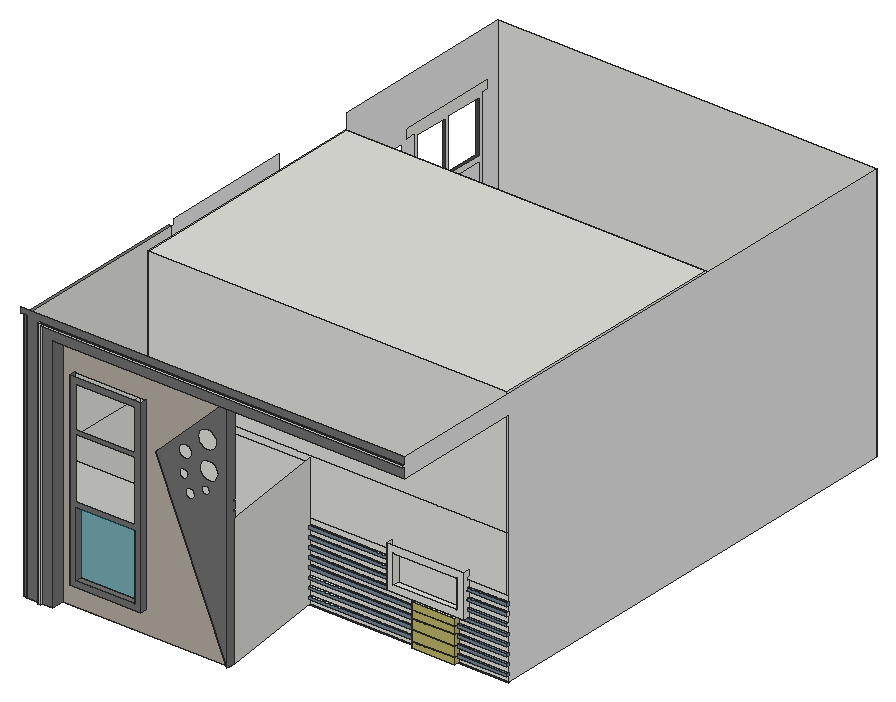
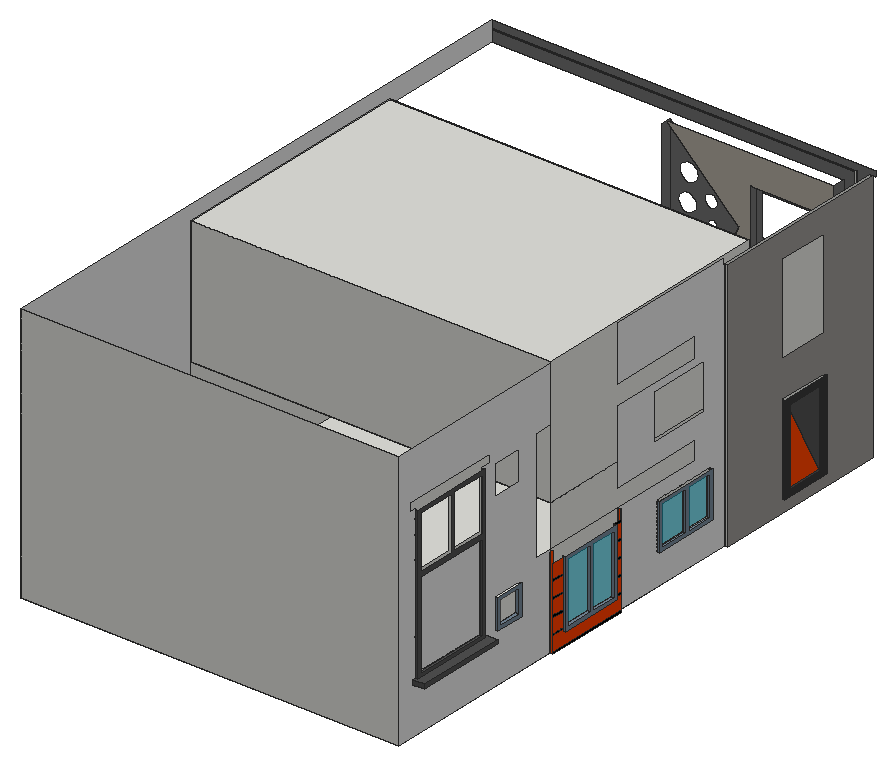
# SketchUp Ruby script. Lengths in inches.
U = 1.inch
M = Sketchup.active_model
def pt(a) = Geom::Point3d.new(a.map { |v| v * U })
def face(e, loops, mat)
  f = e.add_face(loops[0].map { |a| pt(a) })
  loops[1..].each { |l| e.add_face(l.map { |a| pt(a) }).erase! }
  f.material = f.back_material = mat if mat
  f
end
# faces: each face lists its corners as indices into pts; further lists are holes
def faces(e, pts, list, mat = nil) = list.each { |f| face(e, (f[0].is_a?(Array) ? f : [f]).map { |l| l.map { |i| pts[i] } }, mat) }
# xy, xz, yz: faces in a plane at the given z, y or x. An outline is a flat list of corners, or four numbers for a rectangle; further outlines are holes
def ring(l) = l.size == 4 ? [[l[0], l[1]], [l[2], l[1]], [l[2], l[3]], [l[0], l[3]]] : l.each_slice(2).to_a
def flat(e, list, mat, &to3) = list.each { |f| face(e, (f[0].is_a?(Array) ? f : [f]).map { |l| ring(l).map { |u, v| to3.(u, v) } }, mat) }
def xy(e, z, list, mat = nil) = flat(e, list, mat) { |x, y| [x, y, z] }
def xz(e, y, list, mat = nil) = flat(e, list, mat) { |x, z| [x, y, z] }
def yz(e, x, list, mat = nil) = flat(e, list, mat) { |y, z| [x, y, z] }
def lines(e, pts, list) = list.each { |a, b| e.add_line(pt(pts[a]), pt(pts[b])) }
# prism: a flat outline (further loops are holes) pulled along v
def prism(e, loops, v, mat = nil)
  f = face(e, loops, mat); d = Geom::Vector3d.new(v.map { |x| x * U })
  f.pushpull(f.normal.samedirection?(d) ? d.length : -d.length)
end
def box(e, o, s, mat = nil) = prism(e, [[o, [o[0] + s[0], o[1], o[2]], [o[0] + s[0], o[1] + s[1], o[2]], [o[0], o[1] + s[1], o[2]]]], [0, 0, s[2]], mat)
def at(x, y, z, deg = 0) = Geom::Transformation.translation(pt([x, y, z])) * Geom::Transformation.rotation(ORIGIN, Z_AXIS, deg.degrees)
def axes(o, x, y, z) = Geom::Transformation.new([*x, 0, *y, 0, *z, 0, *pt(o).to_a, 1])
def part(name) = M.definitions.add(name)
# library, detail: a bought-in or finely detailed component or shape, given as its bounding box
def library(name, o, s) = part(name).tap { |d| box(d.entities, o, s) }
def detail(e, o, s) = box(e.add_group.entities, o, s)
def put(e, d, t, mat = nil) = e.add_instance(d, t).tap { |i| i.material = mat if mat }
def group(e, t, mat = nil) = e.add_group.tap { |g| g.transformation = t; g.material = mat if mat }.entities
root = M.entities
M.materials.add("[0024_OrangeRed]").color = [255, 69, 0]
M.materials.add("[0057_DarkKhaki]").color = [189, 183, 107]
M.materials.add("[0110_LightSlateGray]").color = [119, 136, 153]
M.materials.add("[0135_DarkGray]").color = [81, 81, 81]
M.materials.add("[Color B05]").color = [255, 63, 0]
M.materials.add("[Color M05]").color = [114, 114, 114]
M.materials.add("[Color M07]").color = [58, 58, 58]
M.materials.add("[Color M09]").color = [0, 0, 0]
M.materials.add("[Concrete Aggregate Smoke]").color = [154, 150, 148]
M.materials.add("[Polished Concrete Old]").color = [229, 229, 229]
M.materials.add("[Stone Masonry Multi]").color = [182, 175, 164]
M.materials.add("[Translucent Glass Gray]").color = [128, 128, 128]
M.materials["[Translucent Glass Gray]"].alpha = 0.5
M.materials.add("[Translucent Glass Tinted]").color = [4, 119, 142]
M.materials["[Translucent Glass Tinted]"].alpha = 0.48
M.materials.add("[Translucent Glass Tinted]1").color = [8, 201, 241]
M.materials["[Translucent Glass Tinted]1"].alpha = 0.48
xy(root,0,[[15,20,18,175.3125],[18,20,18,563,378,563,378,125.9375,27,125.9375,27,20],[27,20,27,125.9375,188.34,125.9375,201.375,20],[15,302.14,18,382.63]])
xy(root,0,[[289.59,120.9375,330.37,125.9375]],"[0057_DarkKhaki]")
xy(root,0,[[30.46,0,30.46,2,18,2,18,20,201.375,20,201.375,14,42.91,14,42.91,2,32.7,2,32.7,0],[15,2,18,20]],"[Color M05]")
xy(root,4.9,[[188.34,123.9375,289.59,125.9375],[330.37,123.9375,363.6875,125.9375],[363.6875,123.9375,378,125.9375]],"[0110_LightSlateGray]")
xy(root,5.67,[[289.59,120.9375,330.37,122.9375]])
xy(root,6.45,[[289.59,120.9375,330.37,122.9375]],"[0057_DarkKhaki]")
xy(root,7.97,[[188.34,123.9375,289.59,125.9375]])
xy(root,7.97,[[330.37,123.9375,378,125.9375]],"[0110_LightSlateGray]")
xy(root,13.12,[[12,60.99,15,110.86]],"[Color M07]")
xy(root,13.47,[[188.34,123.9375,289.59,125.9375],[330.37,123.9375,363.6875,125.9375],[363.6875,123.9375,378,125.9375]],"[0110_LightSlateGray]")
xy(root,15.375,[[12,310.47,15,371.75]],"[0110_LightSlateGray]")
xy(root,15.48,[[289.59,120.9375,330.37,122.9375]])
xy(root,16.27,[[289.59,120.9375,330.37,122.9375]],"[0057_DarkKhaki]")
xy(root,16.53,[[188.34,123.9375,289.59,125.9375]])
xy(root,16.53,[[330.37,123.9375,378,125.9375]],"[0110_LightSlateGray]")
xy(root,18.375,[[12,313.47,15,338.88],[12,341.11,15,368.75]],"[0110_LightSlateGray]")
xy(root,19.12,[[12,66.99,15,104.86]],"[Color M07]")
xy(root,20.43,[[53.9,8,121.9,14]],"[Color M05]")
xy(root,22.03,[[188.34,123.9375,289.59,125.9375],[330.37,123.9375,363.6875,125.9375],[363.6875,123.9375,378,125.9375]],"[0110_LightSlateGray]")
xy(root,25.09,[[188.34,123.9375,289.59,125.9375]])
xy(root,25.09,[[330.37,123.9375,378,125.9375]],"[0110_LightSlateGray]")
xy(root,25.29,[[289.59,120.9375,330.37,122.9375]])
xy(root,26.08,[[289.59,120.9375,330.37,122.9375]],"[0057_DarkKhaki]")
xy(root,26.43,[[59.9,8,115.9,14]],"[Color M05]")
xy(root,30.59,[[188.34,123.9375,289.59,125.9375],[330.37,123.9375,363.6875,125.9375],[363.6875,123.9375,378,125.9375]],"[0110_LightSlateGray]")
xy(root,30.87,[[15,192.9,18,256.21]],"[0110_LightSlateGray]")
xy(root,32.17,[[289.59,120.9375,330.37,122.9375]])
xy(root,32.95,[[289.59,120.9375,330.37,122.9375]],"[0057_DarkKhaki]")
xy(root,33.66,[[188.34,123.9375,289.59,125.9375]])
xy(root,33.66,[[330.37,123.9375,378,125.9375]],"[0110_LightSlateGray]")
xy(root,33.87,[[15,195.9,18,221.52],[15,224.56,18,253.21]],"[0110_LightSlateGray]")
xy(root,39.15,[[289.59,120.9375,330.37,123.9375],[289.59,123.9375,330.37,125.9375]])
xy(root,39.15,[[188.34,123.9375,289.59,125.9375],[330.37,123.9375,363.6875,125.9375],[363.6875,123.9375,378,125.9375]],"[0110_LightSlateGray]")
xy(root,42.22,[[266.69,119.9375,339.4,123.9375],[188.34,123.9375,266.69,125.9375],[266.69,123.9375,339.4,125.9375]])
xy(root,42.22,[[339.4,123.9375,378,125.9375]],"[0110_LightSlateGray]")
xy(root,45.35,[[6,459.92,18,547.29]],"[0135_DarkGray]")
xy(root,47.72,[[188.34,123.9375,266.69,125.9375],[339.4,123.9375,363.6875,125.9375],[363.6875,123.9375,378,125.9375]],"[0110_LightSlateGray]")
xy(root,48.22,[[272.69,119.9375,333.4,125.9375]])
xy(root,48.55,[[15,420.33,18,448.89]],"[0110_LightSlateGray]")
xy(root,49.6,[[15,463.73,18,543.73]])
xy(root,49.6,[[6,459.92,18,459.92,18,463.73,15,463.73,15,543.73,18,543.73,18,547.29,6,547.29]],"[0135_DarkGray]")
xy(root,50.78,[[188.34,123.9375,266.69,125.9375]])
xy(root,50.78,[[339.4,123.9375,378,125.9375]],"[0110_LightSlateGray]")
xy(root,51.55,[[15,423.33,18,445.89]],"[0110_LightSlateGray]")
xy(root,52.6,[[15,466.73,18,540.73]],"[0135_DarkGray]")
xy(root,56.28,[[188.34,123.9375,266.69,125.9375],[339.4,123.9375,363.6875,125.9375],[363.6875,123.9375,378,125.9375]],"[0110_LightSlateGray]")
xy(root,59.34,[[188.34,123.9375,266.69,125.9375]])
xy(root,59.34,[[339.4,123.9375,378,125.9375]],"[0110_LightSlateGray]")
xy(root,64.84,[[188.34,123.9375,266.69,125.9375],[339.4,123.9375,363.6875,125.9375],[363.6875,123.9375,378,125.9375]],"[0110_LightSlateGray]")
xy(root,67.91,[[188.34,123.9375,266.69,125.9375]])
xy(root,67.91,[[339.4,123.9375,378,125.9375]],"[0110_LightSlateGray]")
xy(root,71.62,[[15,195.9,18,221.52],[15,224.56,18,253.21]],"[0110_LightSlateGray]")
xy(root,120,[[27,134.9375,369,371]])
xy(root,240,[[27,134.9375,369,371]])
xz(root,0,[[30.46,0,32.7,0,32.7,238.03,378,238.03,378,239.39,30.46,239.39]])
xz(root,2,[[18,0,30.46,0,30.46,239.39,378,239.39,378,246,12,246,12,240.8125,18,240.8125],[15,0,18,240.8125],[32.7,0,42.91,0,42.91,227.53,378,227.53,378,238.03,32.7,238.03]],"[Color M05]")
xz(root,8,[[[53.9,20.43,121.9,200.12],[59.9,26.43,115.9,89.01],[59.9,93.35,115.9,151.59],[59.9,155.16,115.9,194.12]]],"[Color M05]")
xz(root,11,[[[201.375,0,201.375,227.53,133.54,160.93],[182.83,179.81,180.54,180.11,178.4,181,176.56,182.41,175.15,184.25,174.26,186.39,173.96,188.68,174.26,190.98,175.15,193.12,176.56,194.96,178.4,196.37,180.54,197.26,182.83,197.56,185.13,197.26,187.27,196.37,189.11,194.96,190.52,193.12,191.41,190.98,191.71,188.68,191.41,186.39,190.52,184.25,189.11,182.41,187.27,181,185.13,180.11],[184.53,153.64,182.23,153.94,180.1,154.83,178.27,156.24,176.86,158.07,175.97,160.2,175.67,162.49,175.97,164.79,176.86,166.92,178.27,168.75,180.1,170.16,182.23,171.05,184.53,171.35,186.82,171.05,188.95,170.16,190.79,168.75,192.19,166.92,193.08,164.79,193.38,162.49,193.08,160.2,192.19,158.07,190.79,156.24,188.95,154.83,186.82,153.94],[161.99,165.1,160.37,165.31,158.86,165.93,157.57,166.93,156.58,168.22,155.95,169.73,155.74,171.35,155.95,172.96,156.58,174.47,157.57,175.77,158.86,176.76,160.37,177.38,161.99,177.6,163.61,177.38,165.11,176.76,166.41,175.77,167.4,174.47,168.03,172.96,168.24,171.35,168.03,169.73,167.4,168.22,166.41,166.93,165.11,165.93,163.61,165.31],[166.47,132.54,165.33,132.69,164.28,133.13,163.375,133.83,162.68,134.73,162.24,135.79,162.09,136.92,162.24,138.05,162.68,139.11,163.375,140.01,164.28,140.71,165.33,141.14,166.47,141.29,167.6,141.14,168.65,140.71,169.5625,140.01,170.26,139.11,170.69,138.05,170.84,136.92,170.69,135.79,170.26,134.73,169.5625,133.83,168.65,133.13,167.6,132.69],[160.62,147.68,159.54,147.83,158.53,148.24,157.66,148.91,156.99,149.78,156.58,150.79,156.43,151.87,156.58,152.95,156.99,153.96,157.66,154.83,158.53,155.5,159.54,155.92,160.62,156.06,161.7,155.92,162.71,155.5,163.58,154.83,164.25,153.96,164.67,152.95,164.81,151.87,164.67,150.79,164.25,149.78,163.58,148.91,162.71,148.24,161.7,147.83],[181.03,140.83,180.03,140.97,179.09,141.35,178.29,141.97,177.67,142.77,177.29,143.71,177.15,144.71,177.29,145.71,177.67,146.65,178.29,147.45,179.09,148.0625,180.03,148.45,181.03,148.58,182.03,148.45,182.97,148.0625,183.77,147.45,184.39,146.65,184.77,145.71,184.9,144.71,184.77,143.71,184.39,142.77,183.77,141.97,182.97,141.35,182.03,140.97]]],"[Color M05]")
xz(root,14,[[[42.91,0,201.375,0,133.54,160.93,201.375,227.53,42.91,227.53],[53.9,20.43,121.9,200.12]]],"[Stone Masonry Multi]")
xz(root,14,[[59.9,26.43,115.9,89.01]],"[Translucent Glass Tinted]")
xz(root,20,[[27,0,201.375,120]])
xz(root,60.99,[[12,13.12,15,97.99]],"[Color M07]")
xz(root,66.99,[[12,19.12,15,91.99]],"[Color M07]")
xz(root,104.86,[[12,19.12,15,91.99]],"[Color M07]")
xz(root,110.86,[[12,13.12,15,97.99]],"[Color M07]")
xz(root,119.9375,[[[266.69,42.22,339.4,81.97],[272.69,48.22,333.4,75.97]]])
xz(root,120.9375,[[289.59,0,330.37,5.67],[289.59,6.45,330.37,15.48],[289.59,16.27,330.37,25.29],[289.59,26.08,330.37,32.17],[289.59,32.95,330.37,39.15]],"[0057_DarkKhaki]")
xz(root,122.9375,[[289.59,5.67,330.37,6.45],[289.59,15.48,330.37,16.27],[289.59,25.29,330.37,26.08],[289.59,32.17,330.37,32.95]],"[0057_DarkKhaki]")
xz(root,123.9375,[[188.34,4.9,289.59,7.97],[330.37,4.9,378,7.97],[188.34,13.47,289.59,16.53],[330.37,13.47,378,16.53],[188.34,22.03,289.59,25.09],
  [330.37,22.03,378,25.09],[188.34,30.59,289.59,33.66],[330.37,30.59,378,33.66],[188.34,39.15,378,42.22],[188.34,47.72,266.69,50.78],
  [339.4,47.72,378,50.78],[188.34,56.28,266.69,59.34],[339.4,56.28,378,59.34],[188.34,64.84,266.69,67.91],[339.4,64.84,378,67.91]],"[0110_LightSlateGray]")
xz(root,125.9375,[[188.34,-0.59,378,0],[27,0,188.34,120],[188.34,0,289.59,4.9],[330.37,0,378,4.9],[188.34,4.9,289.59,7.97],
  [330.37,4.9,378,7.97],[188.34,7.97,289.59,13.47],[330.37,7.97,378,13.47],[188.34,13.47,289.59,16.53],[330.37,13.47,378,16.53],
  [188.34,16.53,289.59,22.03],[330.37,16.53,378,22.03],[188.34,22.03,289.59,25.09],[330.37,22.03,378,25.09],[188.34,25.09,289.59,30.59],
  [330.37,25.09,378,30.59],[188.34,30.59,289.59,33.66],[330.37,30.59,378,33.66],[188.34,33.66,289.59,39.15],[330.37,33.66,378,39.15],
  [188.34,39.15,378,42.22],[188.34,42.22,266.69,47.72],[339.4,42.22,378,47.72],[188.34,47.72,266.69,50.78],[272.69,48.22,333.4,75.97],
  [188.34,50.78,266.69,56.28],[339.4,50.78,378,56.28],[188.34,56.28,266.69,59.34],[339.4,56.28,378,59.34],[188.34,59.34,266.69,64.84],
  [339.4,59.34,378,64.84],[188.34,64.84,266.69,67.91],[339.4,64.84,378,67.91],[188.34,67.91,266.69,73.4],[339.4,67.91,378,73.4]])
xz(root,134.9375,[[27,0,369,120],[27,120,369,240]])
xz(root,175.3125,[[15,0,18,240.8125]])
xz(root,192.9,[[15,30.87,18,74.62]],"[0110_LightSlateGray]")
xz(root,195.9,[[15,33.87,18,71.62]],"[0110_LightSlateGray]")
xz(root,221.52,[[15,33.87,18,71.62]],"[0110_LightSlateGray]")
xz(root,224.56,[[15,33.87,18,71.62]],"[0110_LightSlateGray]")
xz(root,253.21,[[15,33.87,18,71.62]],"[0110_LightSlateGray]")
xz(root,256.21,[[15,30.87,18,74.62]],"[0110_LightSlateGray]")
xz(root,302.14,[[15,0,18,88.11]],"[0024_OrangeRed]")
xz(root,310.47,[[12,15.375,15,17.625],[12,17.625,15,79.125]],"[0110_LightSlateGray]")
xz(root,313.47,[[12,18.375,15,76.125]],"[0110_LightSlateGray]")
xz(root,338.88,[[12,18.375,15,76.125]],"[0110_LightSlateGray]")
xz(root,341.11,[[12,18.375,15,76.125]],"[0110_LightSlateGray]")
xz(root,368.75,[[12,18.375,15,76.125]],"[0110_LightSlateGray]")
xz(root,371,[[27,120,369,240]])
xz(root,371.75,[[12,15.375,15,79.125]],"[0110_LightSlateGray]")
xz(root,382.63,[[15,0,18,88.11]],"[0024_OrangeRed]")
xz(root,420.33,[[15,48.55,18,77.11]],"[0110_LightSlateGray]")
xz(root,423.33,[[15,51.55,18,74.11]],"[0110_LightSlateGray]")
xz(root,445.89,[[15,51.55,18,74.11]],"[0110_LightSlateGray]")
xz(root,448.89,[[15,48.55,18,77.11]],"[0110_LightSlateGray]")
xz(root,459.92,[[6,45.35,18,49.6]],"[0135_DarkGray]")
xz(root,463.73,[[15,49.6,18,193.1]],"[0135_DarkGray]")
xz(root,466.73,[[15,52.6,18,135.41]],"[0135_DarkGray]")
xz(root,540.73,[[15,52.6,18,135.41]],"[0135_DarkGray]")
xz(root,543.73,[[15,49.6,18,193.1]],"[0135_DarkGray]")
xz(root,547.29,[[6,45.35,18,49.6]],"[0135_DarkGray]")
xz(root,563,[[18,0,378,246]])
yz(root,6,[[459.92,45.35,547.29,49.6]],"[0135_DarkGray]")
yz(root,12,[[[310.47,15.375,371.75,79.125],[341.11,18.375,368.75,76.125],[313.47,18.375,338.88,76.125]]],"[0110_LightSlateGray]")
yz(root,12,[[[60.99,13.12,110.86,97.99],[66.99,19.12,104.86,91.99]]],"[Color M07]")
yz(root,15,[[66.99,19.12,104.86,91.99,104.86,19.12]],"[0024_OrangeRed]")
yz(root,15,[[[192.9,30.87,256.21,74.62],[224.56,33.87,253.21,71.62],[195.9,33.87,221.52,71.62]],[[420.33,48.55,448.89,77.11],[423.33,51.55,445.89,74.11]]],"[0110_LightSlateGray]")
yz(root,15,[[66.99,19.12,66.99,91.99,104.86,91.99],[[463.73,49.6,543.73,193.1],[466.73,52.6,540.73,135.41],[503.73,139.68,540.73,190.1],[466.73,139.68,500.63,190.1]]],"[0135_DarkGray]")
yz(root,15,[[302.36,2.25,382.63,15.375],[302.36,17.625,310.47,30.75],[371.75,17.625,382.63,30.75],[302.36,33,310.47,46.125],[371.75,33,382.63,46.125],
  [302.36,48.375,310.47,61.5],[371.75,48.375,382.63,61.5],[302.36,63.75,310.47,76.875],[371.75,63.75,382.63,76.875]],"[Color B05]")
yz(root,15,[[302.14,0,302.14,88.11,302.36,88.11,302.36,79.125,310.47,79.125,310.47,76.875,302.36,76.875,302.36,63.75,310.47,63.75,310.47,61.5,302.36,61.5,302.36,48.375,310.47,48.375,310.47,46.125,302.36,46.125,302.36,33,310.47,33,310.47,30.75,302.36,30.75,302.36,17.625,310.47,17.625,310.47,15.375,302.36,15.375,302.36,2.25,382.63,2.25,382.63,0],[371.75,15.375,382.63,17.625],[371.75,30.75,382.63,33],[371.75,46.125,382.63,48.375],[371.75,61.5,382.63,63.75]],"[Color M09]")
yz(root,15,[[[2,0,175.3125,240.8125],[60.99,132.49,110.86,217.37],[60.99,13.12,110.86,97.99]]],"[Concrete Aggregate Smoke]")
yz(root,15,[[313.47,18.375,338.88,76.125],[341.11,18.375,368.75,76.125]],"[Translucent Glass Tinted]1")
yz(root,18,[[2,0,175.3125,240.8125],[302.14,0,382.63,88.11],[[192.9,30.87,256.21,74.62],[224.56,33.87,253.21,71.62],[195.9,33.87,221.52,71.62]],[[463.73,49.6,463.73,193.1,453.79,193.1,453.79,201.17,549.98,201.17,549.98,193.1,543.73,193.1,543.73,49.6],[466.73,52.6,540.73,135.41],[503.73,139.68,540.73,190.1],[466.73,139.68,500.63,190.1]]])
yz(root,18,[[[175.3125,0,175.3125,240.8125,177.0625,240.8125,177.0625,246,302.36,246,302.36,194.23,209.95,194.23,209.95,174.92,302.36,174.92,302.36,105.46,209.95,105.46,209.95,88.11,302.14,88.11,302.14,0],[192.9,30.87,256.21,74.62],[200.12,124.92,258.87,168.42]],[[382.63,0,382.63,88.11,399.82,88.11,399.82,194.23,382.63,194.23,382.63,246,563,246,563,0],[459.92,45.35,547.29,45.35,547.29,49.6,543.73,49.6,543.73,193.1,549.98,193.1,549.98,201.17,453.79,201.17,453.79,193.1,463.73,193.1,463.73,49.6,459.92,49.6],[420.33,161.99,448.89,190.55],[420.33,48.55,448.89,77.11]],[466.73,52.6,540.73,135.41]],"[Polished Concrete Old]")
yz(root,18,[[423.33,51.55,445.89,74.11]],"[Translucent Glass Gray]")
yz(root,18,[[195.9,33.87,221.52,71.62],[224.56,33.87,253.21,71.62]],"[Translucent Glass Tinted]1")
yz(root,27,[[20,0,125.9375,120],[134.9375,0,371,120],[134.9375,120,371,240]])
yz(root,30.46,[[0,0,2,239.39]])
yz(root,32.7,[[0,0,2,238.03]])
yz(root,42.91,[[2,0,14,227.53]],"[Color M05]")
yz(root,53.9,[[8,20.43,14,200.12]],"[Color M05]")
yz(root,59.9,[[8,26.43,14,89.01]],"[Color M05]")
yz(root,115.9,[[8,26.43,14,89.01]],"[Color M05]")
yz(root,121.9,[[8,20.43,14,200.12]],"[Color M05]")
yz(root,188.34,[[123.9375,4.9,125.9375,7.97],[123.9375,13.47,125.9375,16.53],[123.9375,22.03,125.9375,25.09],[123.9375,30.59,125.9375,33.66],[123.9375,39.15,125.9375,42.22],
  [123.9375,47.72,125.9375,50.78],[123.9375,56.28,125.9375,59.34],[123.9375,64.84,125.9375,67.91]])
yz(root,201.375,[[11,0,20,0,20,130.4,18,130.4,18,131.88,20,131.88,20,139.21,18,139.21,18,140.7,20,140.7,20,227.53,11,227.53]],"[Color M05]")
yz(root,266.69,[[119.9375,42.22,119.9375,81.97,125.9375,81.97,125.9375,76.47,123.9375,76.47,123.9375,73.4,125.9375,73.4,125.9375,67.91,123.9375,67.91,123.9375,64.84,125.9375,64.84,125.9375,59.34,123.9375,59.34,123.9375,56.28,125.9375,56.28,125.9375,50.78,123.9375,50.78,123.9375,47.72,125.9375,47.72,125.9375,42.22],[123.9375,47.72,125.9375,50.78],[123.9375,56.28,125.9375,59.34],[123.9375,64.84,125.9375,67.91]])
yz(root,272.69,[[119.9375,48.22,125.9375,75.97]])
yz(root,289.59,[[123.9375,4.9,125.9375,7.97],[123.9375,13.47,125.9375,16.53],[123.9375,22.03,125.9375,25.09],[123.9375,30.59,125.9375,33.66]])
yz(root,289.59,[[120.9375,0,120.9375,5.67,122.9375,5.67,122.9375,6.45,120.9375,6.45,120.9375,15.48,122.9375,15.48,122.9375,16.27,120.9375,16.27,120.9375,25.29,122.9375,25.29,122.9375,26.08,120.9375,26.08,120.9375,32.17,122.9375,32.17,122.9375,32.95,120.9375,32.95,120.9375,39.15,125.9375,39.15,125.9375,33.66,123.9375,33.66,123.9375,30.59,125.9375,30.59,125.9375,25.09,123.9375,25.09,123.9375,22.03,125.9375,22.03,125.9375,16.53,123.9375,16.53,123.9375,13.47,125.9375,13.47,125.9375,7.97,123.9375,7.97,123.9375,4.9,125.9375,4.9,125.9375,0]],"[0057_DarkKhaki]")
yz(root,330.37,[[123.9375,4.9,125.9375,7.97],[123.9375,13.47,125.9375,16.53],[123.9375,22.03,125.9375,25.09],[123.9375,30.59,125.9375,33.66]])
yz(root,330.37,[[120.9375,0,125.9375,0,125.9375,4.9,123.9375,4.9,123.9375,7.97,125.9375,7.97,125.9375,13.47,123.9375,13.47,123.9375,16.53,125.9375,16.53,125.9375,22.03,123.9375,22.03,123.9375,25.09,125.9375,25.09,125.9375,30.59,123.9375,30.59,123.9375,33.66,125.9375,33.66,125.9375,39.15,120.9375,39.15,120.9375,32.95,122.9375,32.95,122.9375,32.17,120.9375,32.17,120.9375,26.08,122.9375,26.08,122.9375,25.29,120.9375,25.29,120.9375,16.27,122.9375,16.27,122.9375,15.48,120.9375,15.48,120.9375,6.45,122.9375,6.45,122.9375,5.67,120.9375,5.67]],"[0057_DarkKhaki]")
yz(root,333.4,[[119.9375,48.22,125.9375,75.97]])
yz(root,339.4,[[119.9375,42.22,125.9375,42.22,125.9375,47.72,123.9375,47.72,123.9375,50.78,125.9375,50.78,125.9375,56.28,123.9375,56.28,123.9375,59.34,125.9375,59.34,125.9375,64.84,123.9375,64.84,123.9375,67.91,125.9375,67.91,125.9375,73.4,123.9375,73.4,123.9375,76.47,125.9375,76.47,125.9375,81.97,119.9375,81.97],[123.9375,56.28,125.9375,59.34],[123.9375,64.84,125.9375,67.91]])
yz(root,369,[[134.9375,0,371,120],[134.9375,120,371,240]])
yz(root,378,[[123.9375,56.28,125.9375,59.34]])
yz(root,378,[[123.9375,4.9,125.9375,7.97],[123.9375,13.47,125.9375,16.53],[123.9375,22.03,125.9375,25.09],[123.9375,30.59,125.9375,33.66],[123.9375,39.15,125.9375,42.22],
  [123.9375,64.84,125.9375,67.91]],"[0110_LightSlateGray]")
yz(root,378,[[125.9375,0,563,0,563,246,2,246,2,239.39,0,239.39,0,238.03,2,238.03,2,227.53,125.9375,227.53,125.9375,50.78,123.9375,50.78,123.9375,47.72,125.9375,47.72]],"[Polished Concrete Old]")
p = [[133.54,14,160.93],[201.375,14,0],[201.375,11,0],[133.54,11,160.93],[201.375,20,0],[188.34,125.9375,0],
  [188.34,125.9375,4.9],[188.34,125.9375,7.97],[188.34,125.9375,13.47],[188.34,125.9375,16.53],[188.34,125.9375,22.03],[188.34,125.9375,25.09],
  [188.34,125.9375,30.59],[188.34,125.9375,33.66],[188.34,125.9375,39.15],[188.34,125.9375,42.22],[188.34,125.9375,47.72],[188.34,125.9375,50.78],
  [188.34,125.9375,56.28],[188.34,125.9375,59.34],[188.34,125.9375,64.84],[188.34,125.9375,67.91],[188.34,125.9375,73.4],[188.34,125.9375,76.47],
  [188.34,125.9375,81.97],[188.34,125.9375,85.03],[188.34,125.9375,90.53],[188.34,125.9375,93.59],[188.34,125.9375,99.09],[188.34,125.9375,102.16],
  [188.34,125.9375,107.65],[188.34,125.9375,110.72],[188.34,125.9375,116.22],[188.34,125.9375,119.28],[188.34,125.9375,120],[188.34,125.9375,124.4375],
  [201.375,20,124.4375],[201.375,20,120]]
faces(root,p,[[0,1,2,3]],"[Color M05]")
faces(root,p,[[4,5,6,7,8,9,10,11,12,13,14,15,16,17,18,19,20,21,22,23,24,25,26,27,28,29,30,31,32,33,34,35,36,37]])
